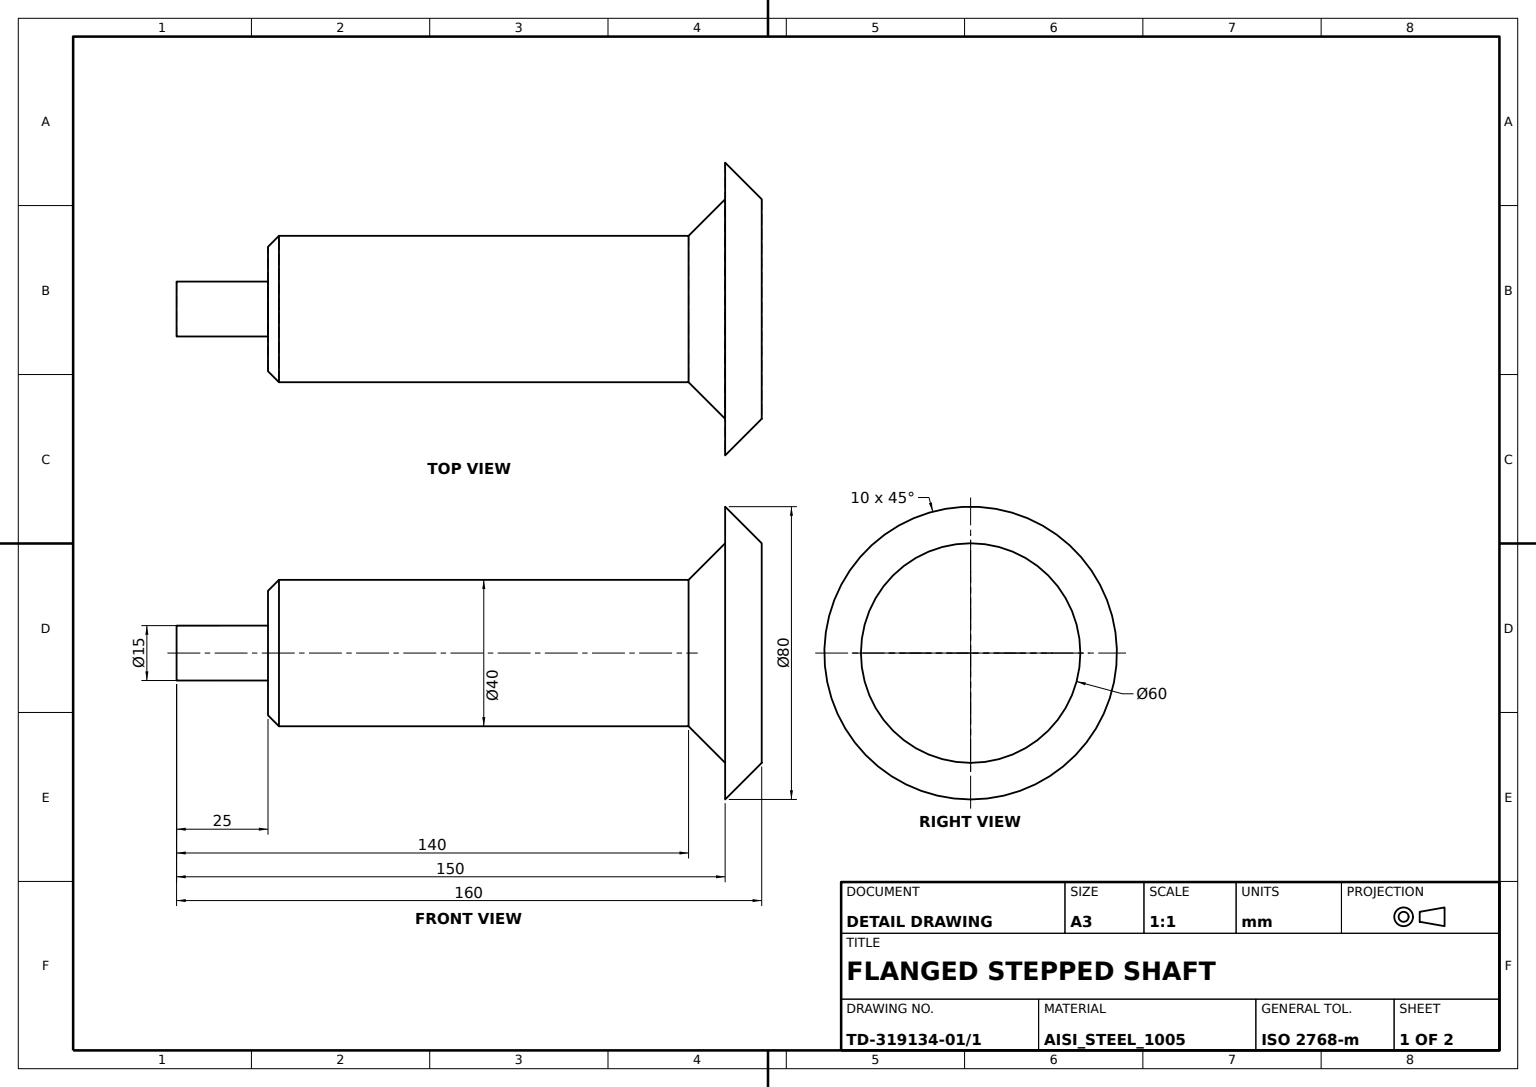
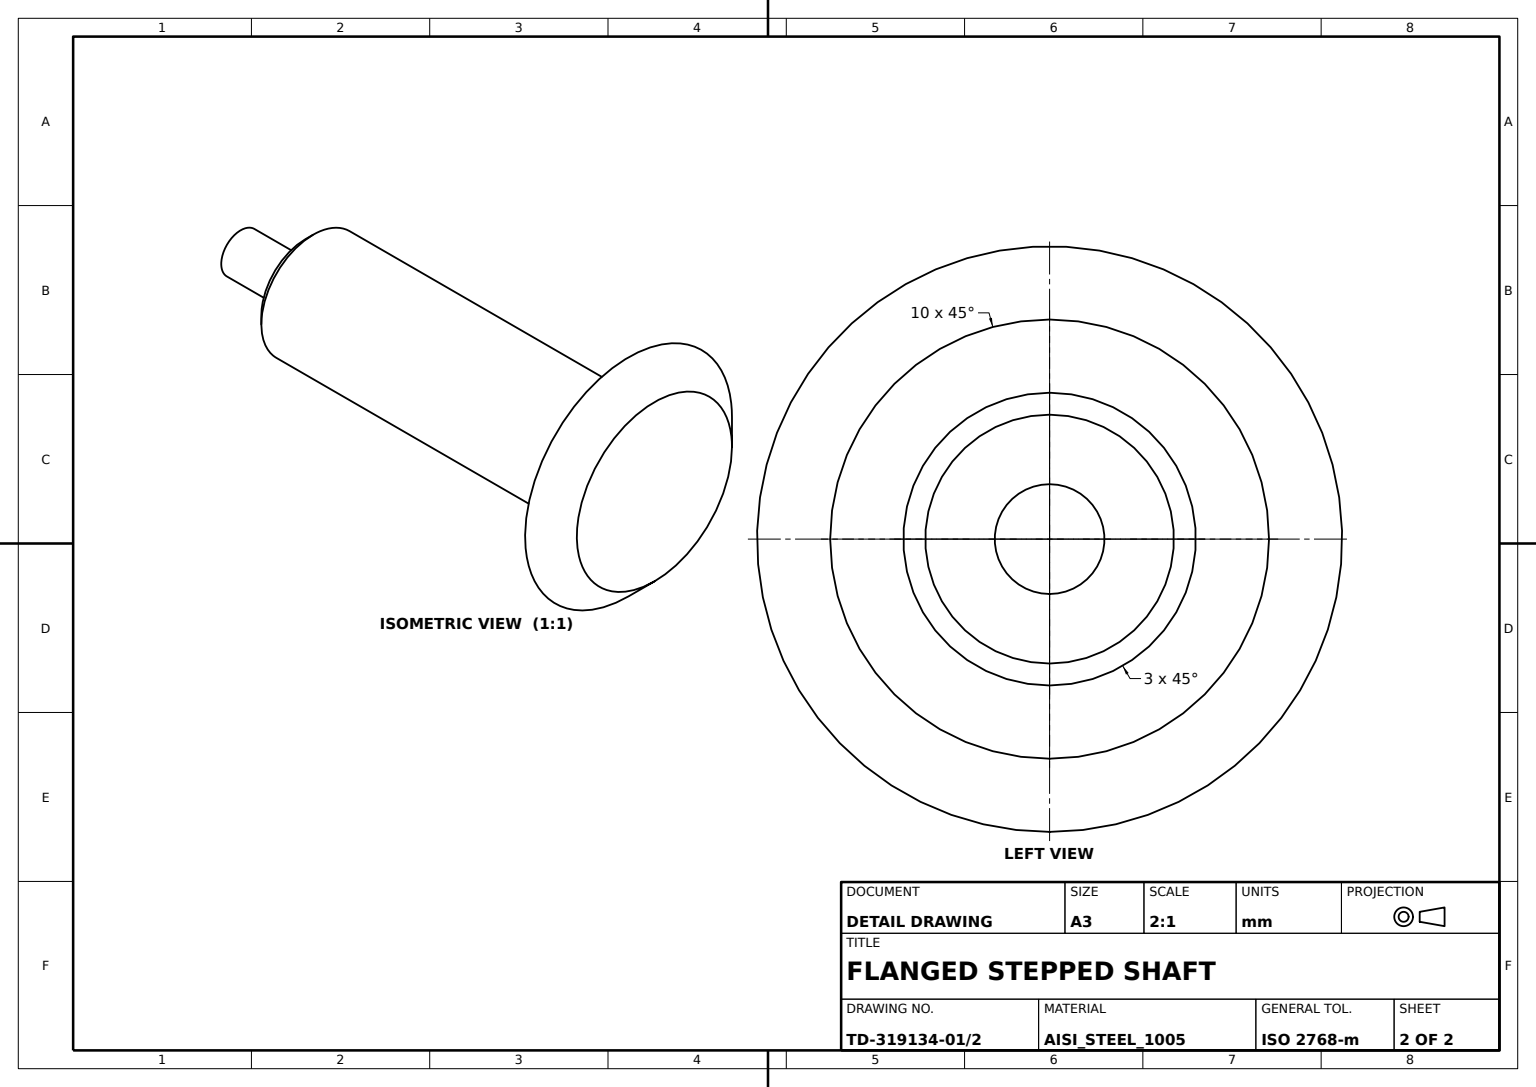
ISO-10303-21;
HEADER;
FILE_DESCRIPTION((''),'2;1');
FILE_NAME('','',(''),(''),'','','');
FILE_SCHEMA(('AUTOMOTIVE_DESIGN'));
ENDSEC;
DATA;
#1=APPLICATION_CONTEXT('');
#2=PRODUCT_CONTEXT('',#1,'mechanical');
#3=PRODUCT('','','',(#2));
#4=PRODUCT_DEFINITION_FORMATION('','',#3);
#5=PRODUCT_DEFINITION_CONTEXT('',#1,'design');
#6=PRODUCT_DEFINITION('','',#4,#5);
#7=PRODUCT_DEFINITION_SHAPE('','',#6);
#8=(LENGTH_UNIT()NAMED_UNIT(*)SI_UNIT(.MILLI.,.METRE.));
#9=(NAMED_UNIT(*)PLANE_ANGLE_UNIT()SI_UNIT($,.RADIAN.));
#10=(NAMED_UNIT(*)SI_UNIT($,.STERADIAN.)SOLID_ANGLE_UNIT());
#11=UNCERTAINTY_MEASURE_WITH_UNIT(LENGTH_MEASURE(0.005),#8,'distance_accuracy_value','');
#12=(GEOMETRIC_REPRESENTATION_CONTEXT(3)GLOBAL_UNCERTAINTY_ASSIGNED_CONTEXT((#11))GLOBAL_UNIT_ASSIGNED_CONTEXT((#8,#9,#10))REPRESENTATION_CONTEXT('',''));
#13=CARTESIAN_POINT('',(0.,38.058252,-20.));
#14=VERTEX_POINT('',#13);
#15=CARTESIAN_POINT('',(0.,38.058252,0.));
#16=DIRECTION('',(0.,-1.,0.));
#17=DIRECTION('',(0.,0.,-1.));
#18=AXIS2_PLACEMENT_3D('',#15,#16,#17);
#19=CIRCLE('',#18,20.);
#20=EDGE_CURVE('',#14,#14,#19,.T.);
#21=ORIENTED_EDGE('',*,*,#20,.F.);
#22=EDGE_LOOP('',(#21));
#23=FACE_BOUND('',#22,.T.);
#24=CARTESIAN_POINT('',(0.,48.058252,-30.));
#25=VERTEX_POINT('',#24);
#26=CARTESIAN_POINT('',(0.,48.058252,0.));
#27=AXIS2_PLACEMENT_3D('',#26,#16,#17);
#28=CIRCLE('',#27,30.);
#29=EDGE_CURVE('',#25,#25,#28,.T.);
#30=ORIENTED_EDGE('',*,*,#29,.T.);
#31=EDGE_LOOP('',(#30));
#32=FACE_BOUND('',#31,.T.);
#33=DIRECTION('',(0.,1.,0.));
#34=DIRECTION('',(0.,0.,1.));
#35=AXIS2_PLACEMENT_3D('',#26,#33,#34);
#36=CONICAL_SURFACE('',#35,30.,0.785398163);
#37=ADVANCED_FACE('',(#23,#32),#36,.T.);
#38=CARTESIAN_POINT('',(0.,-76.941748,17.));
#39=VERTEX_POINT('',#38);
#40=CARTESIAN_POINT('',(0.,-76.941748,0.));
#41=AXIS2_PLACEMENT_3D('',#40,#33,#34);
#42=CIRCLE('',#41,17.);
#43=EDGE_CURVE('',#39,#39,#42,.F.);
#44=ORIENTED_EDGE('',*,*,#43,.F.);
#45=EDGE_LOOP('',(#44));
#46=FACE_BOUND('',#45,.T.);
#47=CARTESIAN_POINT('',(0.,-73.941748,20.));
#48=VERTEX_POINT('',#47);
#49=CARTESIAN_POINT('',(0.,-73.941748,0.));
#50=AXIS2_PLACEMENT_3D('',#49,#33,#34);
#51=CIRCLE('',#50,20.);
#52=EDGE_CURVE('',#48,#48,#51,.T.);
#53=ORIENTED_EDGE('',*,*,#52,.F.);
#54=EDGE_LOOP('',(#53));
#55=FACE_BOUND('',#54,.T.);
#56=CONICAL_SURFACE('',#41,17.,0.785398163);
#57=ADVANCED_FACE('',(#46,#55),#56,.T.);
#58=CARTESIAN_POINT('',(0.,48.058252,-40.));
#59=VERTEX_POINT('',#58);
#60=CIRCLE('',#27,40.);
#61=EDGE_CURVE('',#59,#59,#60,.T.);
#62=ORIENTED_EDGE('',*,*,#61,.F.);
#63=EDGE_LOOP('',(#62));
#64=FACE_BOUND('',#63,.T.);
#65=CARTESIAN_POINT('',(0.,58.058252,-30.));
#66=VERTEX_POINT('',#65);
#67=CARTESIAN_POINT('',(0.,58.058252,0.));
#68=AXIS2_PLACEMENT_3D('',#67,#16,#17);
#69=CIRCLE('',#68,30.);
#70=EDGE_CURVE('',#66,#66,#69,.T.);
#71=ORIENTED_EDGE('',*,*,#70,.T.);
#72=EDGE_LOOP('',(#71));
#73=FACE_BOUND('',#72,.T.);
#74=CONICAL_SURFACE('',#68,30.,0.785398163);
#75=ADVANCED_FACE('',(#64,#73),#74,.T.);
#76=CARTESIAN_POINT('',(0.,-101.941748,-7.5));
#77=VERTEX_POINT('',#76);
#78=CARTESIAN_POINT('',(0.,-101.941748,0.));
#79=AXIS2_PLACEMENT_3D('',#78,#16,#17);
#80=CIRCLE('',#79,7.5);
#81=EDGE_CURVE('',#77,#77,#80,.T.);
#82=ORIENTED_EDGE('',*,*,#81,.T.);
#83=EDGE_LOOP('',(#82));
#84=FACE_BOUND('',#83,.T.);
#85=CARTESIAN_POINT('',(-7.5,-101.941748,0.));
#86=AXIS2_PLACEMENT_3D('',#85,#33,#34);
#87=PLANE('',#86);
#88=ADVANCED_FACE('',(#84),#87,.F.);
#89=ORIENTED_EDGE('',*,*,#70,.F.);
#90=EDGE_LOOP('',(#89));
#91=FACE_BOUND('',#90,.T.);
#92=PLANE('',#68);
#93=ADVANCED_FACE('',(#91),#92,.F.);
#94=ORIENTED_EDGE('',*,*,#20,.T.);
#95=EDGE_LOOP('',(#94));
#96=FACE_BOUND('',#95,.T.);
#97=ORIENTED_EDGE('',*,*,#52,.T.);
#98=EDGE_LOOP('',(#97));
#99=FACE_BOUND('',#98,.T.);
#100=CARTESIAN_POINT('',(0.,0.,0.));
#101=AXIS2_PLACEMENT_3D('',#100,#16,#17);
#102=CYLINDRICAL_SURFACE('',#101,20.);
#103=ADVANCED_FACE('',(#96,#99),#102,.T.);
#104=ORIENTED_EDGE('',*,*,#61,.T.);
#105=EDGE_LOOP('',(#104));
#106=FACE_BOUND('',#105,.T.);
#107=ORIENTED_EDGE('',*,*,#29,.F.);
#108=EDGE_LOOP('',(#107));
#109=FACE_BOUND('',#108,.T.);
#110=CARTESIAN_POINT('',(-40.,48.058252,0.));
#111=AXIS2_PLACEMENT_3D('',#110,#33,#34);
#112=PLANE('',#111);
#113=ADVANCED_FACE('',(#106,#109),#112,.F.);
#114=ORIENTED_EDGE('',*,*,#81,.F.);
#115=EDGE_LOOP('',(#114));
#116=FACE_BOUND('',#115,.T.);
#117=CARTESIAN_POINT('',(0.,-76.941748,-7.5));
#118=VERTEX_POINT('',#117);
#119=AXIS2_PLACEMENT_3D('',#40,#16,#17);
#120=CIRCLE('',#119,7.5);
#121=EDGE_CURVE('',#118,#118,#120,.T.);
#122=ORIENTED_EDGE('',*,*,#121,.T.);
#123=EDGE_LOOP('',(#122));
#124=FACE_BOUND('',#123,.T.);
#125=CYLINDRICAL_SURFACE('',#101,7.5);
#126=ADVANCED_FACE('',(#116,#124),#125,.T.);
#127=ORIENTED_EDGE('',*,*,#121,.F.);
#128=EDGE_LOOP('',(#127));
#129=FACE_BOUND('',#128,.T.);
#130=ORIENTED_EDGE('',*,*,#43,.T.);
#131=EDGE_LOOP('',(#130));
#132=FACE_BOUND('',#131,.T.);
#133=CARTESIAN_POINT('',(-20.,-76.941748,0.));
#134=AXIS2_PLACEMENT_3D('',#133,#33,#34);
#135=PLANE('',#134);
#136=ADVANCED_FACE('',(#129,#132),#135,.F.);
#137=CLOSED_SHELL('',(#37,#57,#75,#88,#93,#103,#113,#126,#136));
#138=MANIFOLD_SOLID_BREP('',#137);
#139=ADVANCED_BREP_SHAPE_REPRESENTATION('',(#138),#12);
#140=SHAPE_DEFINITION_REPRESENTATION(#7,#139);
ENDSEC;
END-ISO-10303-21;
